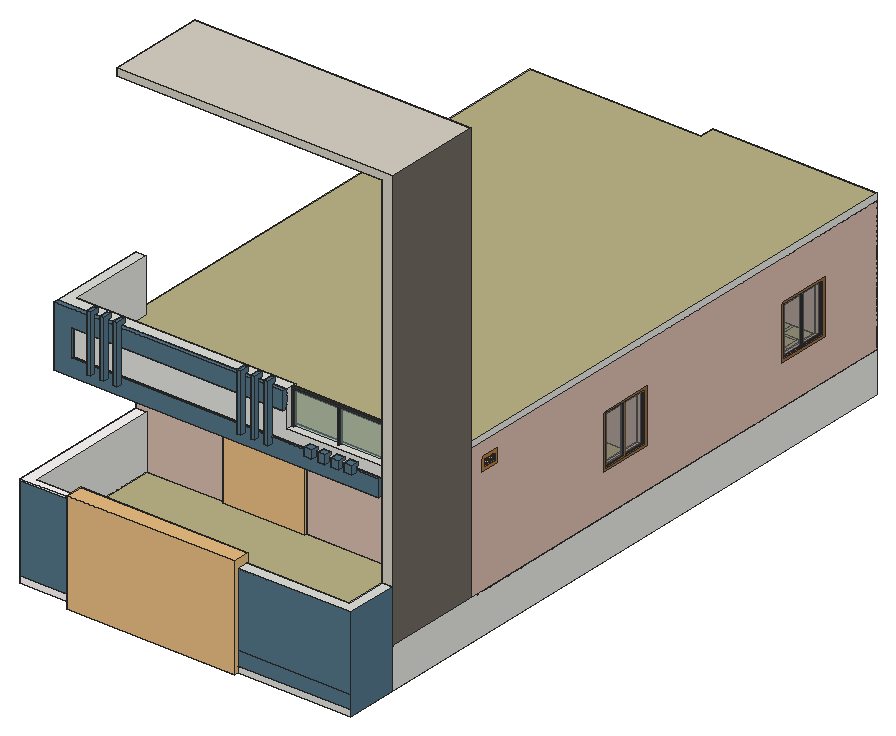
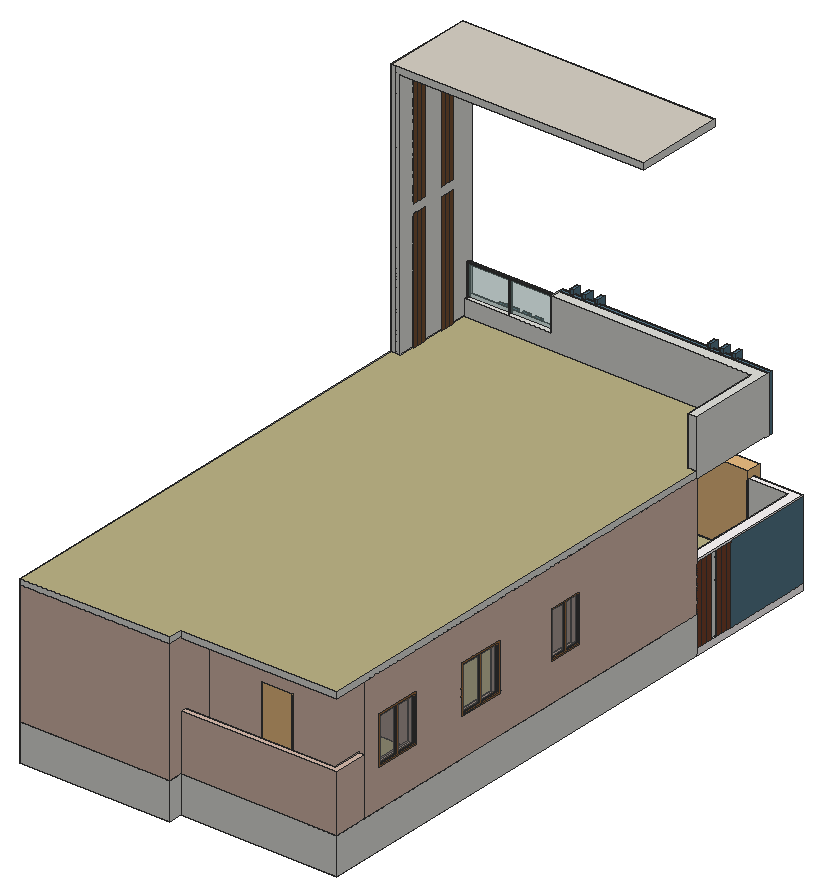
# SketchUp Ruby script. Lengths in inches.
U = 1.inch
M = Sketchup.active_model
def pt(a) = Geom::Point3d.new(a.map { |v| v * U })
def face(e, loops, mat)
  f = e.add_face(loops[0].map { |a| pt(a) })
  loops[1..].each { |l| e.add_face(l.map { |a| pt(a) }).erase! }
  f.material = f.back_material = mat if mat
  f
end
# faces: each face lists its corners as indices into pts; further lists are holes
def faces(e, pts, list, mat = nil) = list.each { |f| face(e, (f[0].is_a?(Array) ? f : [f]).map { |l| l.map { |i| pts[i] } }, mat) }
# xy, xz, yz: faces in a plane at the given z, y or x. An outline is a flat list of corners, or four numbers for a rectangle; further outlines are holes
def ring(l) = l.size == 4 ? [[l[0], l[1]], [l[2], l[1]], [l[2], l[3]], [l[0], l[3]]] : l.each_slice(2).to_a
def flat(e, list, mat, &to3) = list.each { |f| face(e, (f[0].is_a?(Array) ? f : [f]).map { |l| ring(l).map { |u, v| to3.(u, v) } }, mat) }
def xy(e, z, list, mat = nil) = flat(e, list, mat) { |x, y| [x, y, z] }
def xz(e, y, list, mat = nil) = flat(e, list, mat) { |x, z| [x, y, z] }
def yz(e, x, list, mat = nil) = flat(e, list, mat) { |y, z| [x, y, z] }
def lines(e, pts, list) = list.each { |a, b| e.add_line(pt(pts[a]), pt(pts[b])) }
# prism: a flat outline (further loops are holes) pulled along v
def prism(e, loops, v, mat = nil)
  f = face(e, loops, mat); d = Geom::Vector3d.new(v.map { |x| x * U })
  f.pushpull(f.normal.samedirection?(d) ? d.length : -d.length)
end
def box(e, o, s, mat = nil) = prism(e, [[o, [o[0] + s[0], o[1], o[2]], [o[0] + s[0], o[1] + s[1], o[2]], [o[0], o[1] + s[1], o[2]]]], [0, 0, s[2]], mat)
def at(x, y, z, deg = 0) = Geom::Transformation.translation(pt([x, y, z])) * Geom::Transformation.rotation(ORIGIN, Z_AXIS, deg.degrees)
def axes(o, x, y, z) = Geom::Transformation.new([*x, 0, *y, 0, *z, 0, *pt(o).to_a, 1])
def part(name) = M.definitions.add(name)
# library, detail: a bought-in or finely detailed component or shape, given as its bounding box
def library(name, o, s) = part(name).tap { |d| box(d.entities, o, s) }
def detail(e, o, s) = box(e.add_group.entities, o, s)
def put(e, d, t, mat = nil) = e.add_instance(d, t).tap { |i| i.material = mat if mat }
def group(e, t, mat = nil) = e.add_group.tap { |g| g.transformation = t; g.material = mat if mat }.entities
root = M.entities
M.materials.add("TEAKcrown-cut").color = [186, 122, 55]
M.materials.add("[0001_PaleVioletRed]").color = [119, 65, 42]
M.materials.add("[0010_Snow]").color = [255, 250, 250]
M.materials.add("[0027_PeachPuff]").color = [83, 118, 137]
M.materials.add("[0030_OldLace]").color = [216, 209, 197]
M.materials.add("[Carrera Marble]").color = [207, 207, 207]
M.materials.add("[Cladding Weathered]").color = [111, 105, 96]
M.materials.add("[Color B01]").color = [216, 187, 172]
M.materials.add("[Color E03]").color = [255, 255, 101]
M.materials.add("[Color E05]").color = [255, 255, 0]
M.materials.add("[Color M07]").color = [58, 58, 58]
M.materials.add("[Field Rectangle Tile]").color = [193, 186, 176]
M.materials.add("[Sandstone]").color = [118, 81, 52]
M.materials.add("[Stone Marble]").color = [143, 138, 136]
M.materials.add("[Tile Ceramic Natural]").color = [189, 180, 134]
M.materials.add("[Translucent Glass Blue]").color = [141, 178, 174]
M.materials["[Translucent Glass Blue]"].alpha = 0.5
M.materials.add("[Translucent Glass Gray]").color = [128, 128, 128]
M.materials["[Translucent Glass Gray]"].alpha = 0.5
M.materials.add("[Translucent_Glass_Gray]3").color = [255, 255, 255]
M.materials["[Translucent_Glass_Gray]3"].alpha = 0.5
M.materials.add("[Wood Bamboo]").color = [122, 73, 29]
M.materials.add("[Wood Cherry Original]").color = [152, 86, 42]
M.materials.add("[Wood Floor]").color = [155, 105, 61]
c1 = library("Group\#41",[0,0,0],[150.05,15.22,91.0625])
c2 = part("Timber upright")
xy(c2.entities,0,[[0,0,2,5.09]],"[0001_PaleVioletRed]")
xy(c2.entities,76.5,[[0,0,2,5.09]],"[0001_PaleVioletRed]")
xz(c2.entities,0,[[0,0,2,76.5]])
xz(c2.entities,5.09,[[0,0,2,76.5]],"[0001_PaleVioletRed]")
yz(c2.entities,0,[[0,0,5.09,76.5]],"[0001_PaleVioletRed]")
yz(c2.entities,2,[[0,0,5.09,76.5]],"[0001_PaleVioletRed]")
c3 = part("Timber slat")
box(c3.entities,[0,37.3125,0],[3.6875,119.625,1.02],"[Sandstone]")
c4 = part("Group\#44")
put(c4.entities,c3,at(9.375,-37.3125,0))
put(c4.entities,c3,at(4.6875,-37.3125,0))
put(c4.entities,c3,at(0,-37.3125,0))
c5 = library("door by lz",[5.91,-4.92,0],[35.43,6.61,78.74])
c6 = part("Component\#10")
box(c6.entities,[0,0,0],[19,0.25,3.7],"[Translucent_Glass_Gray]3")
c7 = part("Ventilation_window")
g1 = group(c7.entities,at(-76.91,6.38,0),"TEAKcrown-cut")
xy(g1,-1.7,[[0,0,24,3]])
xy(g1,2.5,[[2.5,0,21.5,3]])
xy(g1,17.5,[[2.5,0,21.5,3]])
xy(g1,21.7,[[0,0,24,3]])
xz(g1,0,[[[0,-1.7,24,21.7],[2.5,2.5,21.5,17.5]]],"TEAKcrown-cut")
xz(g1,3,[[[0,-1.7,24,21.7],[2.5,2.5,21.5,17.5]]])
yz(g1,0,[[0,-1.7,3,21.7]])
yz(g1,2.5,[[0,2.5,3,2.5,3,4.31,0,6.48],[3,4.31,3,17.5,0,17.5,0,6.48]])
yz(g1,21.5,[[0,2.5,3,17.5]])
yz(g1,24,[[0,-1.7,3,21.7]])
put(g1,c6,axes([2.5,3.14,11.94],[1,0,0],[0,0.58779,0.80902],[0,-0.80902,0.58779]))
put(g1,c6,axes([2.5,3.16,14.6],[1,0,0],[0,0.58779,0.80902],[0,-0.80902,0.58779]))
put(g1,c6,axes([2.5,3,4.31],[1,0,0],[0,0.58779,0.80902],[0,-0.80902,0.58779]))
put(g1,c6,axes([2.5,3.14,9.46],[1,0,0],[0,0.58779,0.80902],[0,-0.80902,0.58779]))
put(g1,c6,axes([2.5,2.99,7.08],[1,0,0],[0,0.58779,0.80902],[0,-0.80902,0.58779]))
c8 = part("window full")
xy(c8.entities,0,[[0,0,14.17,66.54]])
xy(c8.entities,2.26,[[12.2,2.26,14.17,64.28]],"[Wood Floor]")
xy(c8.entities,2.36,[[0,2.36,1.97,64.17]],"[Wood Floor]")
xy(c8.entities,3.74,[[11.42,3.74,12.2,32.875],[11.42,33.66,12.2,62.79]],"[Wood Floor]")
xy(c8.entities,3.9375,[[1.97,3.9375,2.76,32.77],[1.97,33.76,2.76,62.6]],"[Wood Floor]")
xy(c8.entities,4.18,[[2.76,4.18,11.42,32.09],[2.76,34.45,11.42,62.35]],"[Wood Floor]")
xy(c8.entities,69.83,[[2.76,4.18,11.42,32.09],[2.76,34.45,11.42,62.35]],"[Wood Floor]")
xy(c8.entities,70.08,[[1.97,3.9375,2.76,32.77],[1.97,33.76,2.76,62.6]])
xy(c8.entities,70.27,[[11.42,32.875,12.2,33.66]])
xy(c8.entities,70.27,[[11.42,3.74,12.2,32.875],[11.42,33.66,12.2,62.79]],"[Wood Floor]")
xy(c8.entities,71.65,[[0,2.36,1.97,64.17]])
xy(c8.entities,71.76,[[12.2,2.26,14.17,64.28]],"[Wood Floor]")
xy(c8.entities,74.02,[[0,0,14.17,66.54]],"[Wood Floor]")
xz(c8.entities,0,[[0,0,14.17,74.02]],"[Wood Floor]")
xz(c8.entities,2.26,[[12.2,2.26,14.17,71.76]],"[Wood Floor]")
xz(c8.entities,2.36,[[0,2.36,1.97,71.65]],"[Wood Floor]")
xz(c8.entities,3.74,[[11.42,3.74,12.2,70.27]],"[Wood Floor]")
xz(c8.entities,3.9375,[[1.97,3.9375,2.76,70.08]],"[Wood Floor]")
xz(c8.entities,4.18,[[2.76,4.18,11.42,69.83]],"[Wood Floor]")
xz(c8.entities,32.09,[[2.76,4.18,11.42,69.83]],"[Wood Floor]")
xz(c8.entities,32.77,[[1.97,3.9375,2.76,70.08]],"[Wood Floor]")
xz(c8.entities,32.875,[[11.42,3.74,12.2,70.27]],"[Wood Floor]")
xz(c8.entities,33.66,[[11.42,3.74,12.2,47.88],[11.42,47.88,12.2,70.27]],"[Wood Floor]")
xz(c8.entities,33.76,[[1.97,3.9375,2.76,70.08]],"[Wood Floor]")
xz(c8.entities,34.45,[[2.76,4.18,11.42,69.83]],"[Wood Floor]")
xz(c8.entities,62.35,[[2.76,4.18,11.42,69.83]],"[Wood Floor]")
xz(c8.entities,62.6,[[1.97,3.9375,2.76,70.08]],"[Wood Floor]")
xz(c8.entities,62.79,[[11.42,3.74,12.2,70.27]],"[Wood Floor]")
xz(c8.entities,64.17,[[0,2.36,1.97,71.65]],"[Wood Floor]")
xz(c8.entities,64.28,[[12.2,2.26,14.17,71.76]],"[Wood Floor]")
xz(c8.entities,66.54,[[0,0,14.17,74.02]],"[Wood Floor]")
yz(c8.entities,0,[[[0,0,66.54,74.02],[2.36,2.36,64.17,71.65]]],"[Wood Floor]")
yz(c8.entities,1.97,[[[2.36,2.36,64.17,71.65],[3.9375,3.9375,32.77,70.08],[33.76,3.9375,62.6,70.08]]],"[Wood Floor]")
yz(c8.entities,2.76,[[32.77,3.9375,33.76,4.18],[32.77,4.18,33.76,69.83],[32.77,69.83,33.76,70.08]])
yz(c8.entities,2.76,[[[3.9375,3.9375,32.77,70.08],[4.18,4.18,32.09,69.83]],[[33.76,3.9375,62.6,70.08],[34.45,4.18,62.35,69.83]]],"[Wood Floor]")
yz(c8.entities,11.42,[[32.875,69.83,33.66,70.27]])
yz(c8.entities,11.42,[[[3.74,3.74,32.875,70.27],[4.18,4.18,32.09,69.83]],[[33.66,3.74,62.79,70.27],[34.45,4.18,62.35,69.83]]],"[Wood Floor]")
yz(c8.entities,12.2,[[[2.26,2.26,64.28,71.76],[3.74,3.74,32.875,70.27],[33.66,3.74,62.79,70.27]]],"[Wood Floor]")
yz(c8.entities,14.17,[[[0,0,66.54,74.02],[2.26,2.26,64.28,71.76]]],"[Wood Floor]")
p = [[11.42,32.875,70.27],[11.42,32.875,70.28],[11.42,32.875,69.83],[11.42,32.09,69.83],[11.42,34.45,69.83],[11.42,33.66,69.83]]
lines(c8.entities,p,[[0,1],[2,3],[4,5]])
c9 = part("Group\#7")
g2 = group(c9.entities,at(1.67,3.02,2.71))
yz(g2,0,[[0,0,20.13,42.58]],"[Translucent Glass Gray]")
g3 = group(c9.entities,at(0,0,0))
put(g3,c8,axes([0,0,0],[0.2352,0,0],[0,0.72142,0],[0,0,0.64851]))
g4 = group(g3,at(1.67,24.85,2.71))
yz(g4,0,[[0,0,20.13,42.58]],"[Translucent Glass Gray]")
c10 = part("Group30\#1")
xy(c10.entities,0,[[-14.0625,-20.0625,-0.59,20.0625],[0.59,-20.0625,14.0625,20.0625]],"[Translucent Glass Gray]")
c11 = part("Group29\#1")
prism(c11.entities,[[[-18,24,0],[18,24,0],[18,-24,0],[-18,-24,0]],[[14.0625,20.0625,0],[0.59,20.0625,0],[0.59,-20.0625,0],[14.0625,-20.0625,0]],[[-0.59,20.0625,0],[-14.0625,20.0625,0],[-14.0625,-20.0625,0],[-0.59,-20.0625,0]]],[0,0,5.875],"[Wood Cherry Original]")
put(c11.entities,c10,at(0,0,2.9375))
c12 = part("Union\#2")
xy(c12.entities,0,[[0,87.5,0,494.5,71.05,494.5,71.05,485.5,9,485.5,9,387.5,117,387.5,117,381.5,9,381.5,9,213.5,113.3,213.5,113.3,207.5,9,207.5,9,93.5,79.73,93.5,79.73,87.5],[[153,87.5,153,93.5,239,93.5,239,171.5,153,171.5,153,207.5,143.3,207.5,143.3,213.5,153,213.5,153,286.45,159,286.45,159,177.5,250.23,177.5,250.23,171.5,245,171.5,245,93.5,291,93.5,291,171.5,274.23,171.5,274.23,177.5,291,177.5,291,321.5,159,321.5,159,316.45,153,316.45,153,347.3125,159,347.3125,159,327.5,246,327.5,246,383.5,159,383.5,159,389.5,291,389.5,291,533.5,159,533.5,159,424.27,153,424.27,153,431.5,144.37,431.5,144.37,437.5,153,437.5,153,485.5,117,485.5,117,437.5,124.37,437.5,124.37,431.5,117,431.5,117,424.23,111,424.23,111,485.5,101.05,485.5,101.05,494.5,153,494.5,153,542.5,300,542.5,300,87.5],[252,327.5,291,383.5]],[153,377.3125,158.97,394.27],[111,387.5,117,394.27]])
xy(c12.entities,36,[[250.39,87.5,286.39,93.5],[0,230.6875,9,266.6875],[291,236.77,300,284.77],[0,328.61,9,376.61],[0,430.49,9,478.49],
  [291,436.51,300,484.51]])
xy(c12.entities,84,[[250.39,87.5,286.39,93.5],[250.23,171.5,274.23,177.5],[113.3,207.5,143.3,213.5],[0,230.6875,9,266.6875],[291,236.77,300,284.77],
  [153,286.45,159,316.45],[0,328.61,9,376.61],[153,347.3125,158.97,377.3125],[111,394.27,117,424.23],[153,394.27,159,424.27],
  [0,430.49,9,478.49],[124.37,431.5,144.37,437.5],[291,436.51,300,484.51],[71.05,485.5,101.05,494.5]])
xy(c12.entities,96,[[291,100.54,300,117.47]])
xy(c12.entities,108,[[291,100.54,300,117.47]])
xy(c12.entities,120,[[[0,87.5,79.73,87.5,79.73,93.5,9,93.5,9,207.5,153,207.5,153,171.5,239,171.5,239,93.5,153,93.5,153,87.5,300,87.5,300,542.5,153,542.5,153,494.5,0,494.5],[9,213.5,9,381.5,117,381.5,117,431.5,153,431.5,153,213.5],[159,327.5,159,347.3125,158.97,347.3125,158.97,394.27,159,394.27,159,533.5,291,533.5,291,389.5,159,389.5,159,383.5,246,383.5,246,327.5],[159,177.5,291,321.5],[9,387.5,111,485.5],[245,93.5,291,171.5],[252,327.5,291,383.5],[117,437.5,153,485.5]]])
xz(c12.entities,87.5,[[0,0,79.73,120],[[153,0,300,120],[250.39,36,286.39,84]]])
xz(c12.entities,93.5,[[9,0,79.73,120],[153,0,239,120],[[245,0,291,120],[250.39,36,286.39,84]]])
xz(c12.entities,100.54,[[291,96,300,108]])
xz(c12.entities,117.47,[[291,96,300,108]])
xz(c12.entities,171.5,[[153,0,239,120],[245,0,250.23,0,250.23,84,274.23,84,274.23,0,291,0,291,120,245,120]])
xz(c12.entities,177.5,[[159,0,159,120,291,120,291,0,274.23,0,274.23,84,250.23,84,250.23,0]])
xz(c12.entities,207.5,[[9,0,113.3,0,113.3,84,143.3,84,143.3,0,153,0,153,120,9,120]])
xz(c12.entities,213.5,[[9,0,113.3,120],[143.3,0,143.3,84,113.3,84,113.3,120,153,120,153,0]])
xz(c12.entities,230.6875,[[0,36,9,84]])
xz(c12.entities,236.77,[[291,36,300,84]])
xz(c12.entities,266.6875,[[0,36,9,84]])
xz(c12.entities,284.77,[[291,36,300,84]])
xz(c12.entities,286.45,[[153,0,159,84]])
xz(c12.entities,316.45,[[153,0,159,84]])
xz(c12.entities,321.5,[[159,0,291,120]])
xz(c12.entities,327.5,[[159,0,246,120],[252,0,291,120]])
xz(c12.entities,328.61,[[0,36,9,84]])
xz(c12.entities,347.3125,[[153,0,153,84,158.97,84,158.97,120,159,120,159,0]])
xz(c12.entities,376.61,[[0,36,9,84]])
xz(c12.entities,377.3125,[[153,0,158.97,84]])
xz(c12.entities,381.5,[[9,0,117,120]])
xz(c12.entities,383.5,[[159,0,246,120],[252,0,291,120]])
xz(c12.entities,387.5,[[9,0,111,120]])
xz(c12.entities,389.5,[[159,0,291,120]])
xz(c12.entities,394.27,[[111,0,117,84],[153,0,158.97,84],[158.97,84,159,120]])
xz(c12.entities,424.23,[[111,0,117,84]])
xz(c12.entities,424.27,[[153,0,159,84]])
xz(c12.entities,430.49,[[0,36,9,84]])
xz(c12.entities,431.5,[[117,0,124.37,0,124.37,84,144.37,84,144.37,0,153,0,153,120,117,120]])
xz(c12.entities,436.51,[[291,36,300,84]])
xz(c12.entities,437.5,[[117,0,117,120,153,120,153,0,144.37,0,144.37,84,124.37,84,124.37,0]])
xz(c12.entities,478.49,[[0,36,9,84]])
xz(c12.entities,484.51,[[291,36,300,84]])
xz(c12.entities,485.5,[[9,0,71.05,0,71.05,84,101.05,84,101.05,0,111,0,111,120,9,120],[117,0,153,120]])
xz(c12.entities,494.5,[[0,0,0,120,153,120,153,0,101.05,0,101.05,84,71.05,84,71.05,0]])
xz(c12.entities,533.5,[[159,0,291,120]])
xz(c12.entities,542.5,[[153,0,300,120]])
yz(c12.entities,0,[[[87.5,0,494.5,120],[430.49,36,478.49,84],[328.61,36,376.61,84],[230.6875,36,266.6875,84]]])
yz(c12.entities,9,[[93.5,0,207.5,120],[[213.5,0,381.5,120],[328.61,36,376.61,84],[230.6875,36,266.6875,84]],[[387.5,0,485.5,120],[430.49,36,478.49,84]]])
yz(c12.entities,71.05,[[485.5,0,494.5,84]])
yz(c12.entities,79.73,[[87.5,0,93.5,120]])
yz(c12.entities,101.05,[[485.5,0,494.5,84]])
yz(c12.entities,111,[[387.5,0,387.5,120,485.5,120,485.5,0,424.23,0,424.23,84,394.27,84,394.27,0]])
yz(c12.entities,113.3,[[207.5,0,213.5,84]])
yz(c12.entities,117,[[381.5,0,394.27,0,394.27,84,424.23,84,424.23,0,431.5,0,431.5,120,381.5,120],[437.5,0,485.5,120]])
yz(c12.entities,124.37,[[431.5,0,437.5,84]])
yz(c12.entities,143.3,[[207.5,0,213.5,84]])
yz(c12.entities,144.37,[[431.5,0,437.5,84]])
yz(c12.entities,153,[[87.5,0,93.5,120],[171.5,0,207.5,120],[213.5,0,213.5,120,431.5,120,431.5,0,424.27,0,424.27,84,394.27,84,394.27,0,377.3125,0,377.3125,84,347.3125,84,347.3125,0,316.45,0,316.45,84,286.45,84,286.45,0],[437.5,0,485.5,120],[494.5,0,542.5,120]])
yz(c12.entities,158.97,[[377.3125,0,394.27,0,394.27,120,347.3125,120,347.3125,84,377.3125,84]])
yz(c12.entities,159,[[177.5,0,286.45,0,286.45,84,316.45,84,316.45,0,321.5,0,321.5,120,177.5,120],[327.5,0,347.3125,120],[383.5,0,389.5,120],[424.27,0,533.5,0,533.5,120,394.27,120,394.27,84,424.27,84]])
yz(c12.entities,239,[[93.5,0,171.5,120]])
yz(c12.entities,245,[[93.5,0,171.5,120]])
yz(c12.entities,246,[[327.5,0,383.5,120]])
yz(c12.entities,250.23,[[171.5,0,177.5,84]])
yz(c12.entities,250.39,[[87.5,36,93.5,84]])
yz(c12.entities,252,[[327.5,0,383.5,120]])
yz(c12.entities,274.23,[[171.5,0,177.5,84]])
yz(c12.entities,286.39,[[87.5,36,93.5,84]])
yz(c12.entities,291,[[[93.5,0,171.5,120],[100.54,96,117.47,108]],[[177.5,0,321.5,120],[236.77,36,284.77,84]],[327.5,0,383.5,120],[[389.5,0,533.5,120],[436.51,36,484.51,84]]])
yz(c12.entities,300,[[[87.5,0,542.5,120],[436.51,36,484.51,84],[236.77,36,284.77,84],[100.54,96,117.47,108]]])
put(c12.entities,c5,axes([153.59,321.46,0],[0,-0.84667,0],[0.14881,0,0],[0,0,1.0668]))
put(c12.entities,c5,axes([153.59,382.32,0],[0,-0.84667,0],[0.14881,0,0],[0,0,1.0668]))
put(c12.entities,c5,axes([153.59,429.27,0],[0,-0.84667,0],[0.14881,0,0],[0,0,1.0668]))
put(c12.entities,c5,axes([116.41,429.27,0],[0,-0.84667,0],[-0.14881,0,0],[0,0,1.0668]))
put(c12.entities,c5,axes([108.3,208.09,0],[0.84667,0,0],[0,0.14881,0],[0,0,1.0668]))
put(c12.entities,c5,axes([246.23,177.5,0],[0.67733,0,0],[0,0.14881,0],[0,0,1.0668]))
put(c12.entities,c5,axes([66.05,494.59,0],[0.84667,0,0],[0,0.14881,0],[0,0,1.0668]))
put(c12.entities,c7,axes([303.45,154.81,96.87],[0,0.70573,0],[-0.54,0,0],[0,0,0.51282]))
put(c12.entities,c9,at(0,328.61,36))
put(c12.entities,c9,at(0,430.49,36))
put(c12.entities,c9,at(296.67,436.51,36))
put(c12.entities,c9,at(296.67,236.77,36))
put(c12.entities,c9,axes([0,230.6875,36],[1,0,0],[0,0.75,0],[0,0,1]))
put(c12.entities,c11,axes([268.39,93.375,60],[1,0,0],[0,0,1],[0,-1,0]))
c13 = library("Group\#49",[0,0,0],[78.74,4.71,80.71])
c14 = part("Bed - Queen")
p = [[22,23.6,0],[16.8,23.6,0],[22,38.8,0],[1.2,38.8,0],[1.2,25.6,0],[-1.2,38.8,0],
  [-1.2,25.6,0],[-22,38.8,0],[-22,25.6,0],[30,-40,0],[-30,-40,0],[-30,40,0],
  [14.8,23.2,0],[-30,23.2,0],[-30,25.6,0],[14.8,25.6,0],[30,40,0],[30,10.4,0],
  [14.8,10.4,0]]
lines(c14.entities,p,[[0,1],[2,0],[3,2],[4,3],[5,6],[7,5],[8,7],[9,10],[10,11],[12,13],[14,15],[11,16],
  [16,9],[17,15],[18,17],[15,18]])
c15 = library("*U5",[-21.75,-46.5,0],[21,33,0.01])
c16 = part("*U1")
p = [[-20,-17,0],[-20,23,0],[-18.25,23,0],[-18.25,-17,0],[20,-17,0],[19.92,-14.49,0],
  [19.68,-11.99,0],[19.29,-9.5,0],[18.74,-7.05,0],[18.04,-4.64,0],[17.19,-2.28,0],[16.19,0.03,0],
  [15.05,2.27,0],[13.77,4.43,0],[12.36,6.51,0],[10.82,8.5,0],[9.16,10.38,0],[7.38,12.16,0],
  [5.5,13.82,0],[3.51,15.36,0],[1.43,16.77,0],[-0.73,18.05,0],[-2.97,19.19,0],[-5.28,20.19,0],
  [-7.64,21.04,0],[-10.05,21.74,0],[-12.5,22.29,0],[-14.99,22.68,0],[-17.49,22.92,0],[-20,-23,0],
  [20,-23,0]]
lines(c16.entities,p,[[0,1],[1,2],[2,3],[3,0],[4,5],[5,6],[6,7],[7,8],[8,9],[9,10],[10,11],[11,12],
  [12,13],[13,14],[14,15],[15,16],[16,17],[17,18],[18,19],[19,20],[20,21],[21,22],[22,23],[23,24],
  [24,25],[25,26],[26,27],[27,28],[28,1],[0,29],[4,30]])
c17 = library("SINK",[-14.49,-22.42,0],[28.98,44.84,0.01])
c18 = library("new block",[-14.35,-4.62,0],[28.7,9.24,0.01])
c19 = part("Union\#4")
prism(c19.entities,[[[153,29,0],[6,29,0],[6,0,0],[0,0,0],[0,35,0],[153,35,0]]],[0,0,55.4375])
c20 = library("Group\#3",[0,0,0],[86,78,119.99])
c21 = part("Component\#9")
xy(c21.entities,0,[[[0,0,6.875,4],[0.7,0.7,6.17,3.3]]],"[Color E05]")
xy(c21.entities,0.625,[[0.7,0.7,6.17,3.3]],"[Color E05]")
xy(c21.entities,4.5625,[[0,4,6.875,6.6875]])
xy(c21.entities,7.25,[[0,0,6.875,6.6875]],"[0027_PeachPuff]")
xz(c21.entities,0,[[0,0,6.875,7.25]],"[0027_PeachPuff]")
xz(c21.entities,0.7,[[0.7,0,6.17,0.625]])
xz(c21.entities,3.3,[[0.7,0,6.17,0.625]],"[Color E05]")
xz(c21.entities,4,[[0,0,6.875,4.5625]])
xz(c21.entities,6.6875,[[0,4.5625,6.875,7.25]])
yz(c21.entities,0,[[0,0,0,7.25,6.6875,7.25,6.6875,4.5625,4,4.5625,4,0]],"[0027_PeachPuff]")
yz(c21.entities,0.7,[[0.7,0,3.3,0.625]],"[Color E05]")
yz(c21.entities,6.17,[[0.7,0,3.3,0.625]],"[Color E05]")
yz(c21.entities,6.875,[[0,0,4,0,4,4.5625,6.6875,4.5625,6.6875,7.25,0,7.25]],"[0027_PeachPuff]")
c22 = part("Vertical support post")
prism(c22.entities,[[[3.5625,0,-4],[3.5625,0,43.375],[3.5625,4,43.375],[3.5625,4,47.375],[3.5625,-4,47.375],[3.5625,-4,-4]]],[-3.5625,0,0],"[0027_PeachPuff]")
c23 = part("Group70\#1")
box(c23.entities,[313.8,73.72,268.25],[1.18,2.36,29.23])
c24 = part("Group69\#1")
box(c24.entities,[356.12,73.72,268.25],[2.36,2.36,29.23])
c25 = part("Group71\#1")
box(c25.entities,[270.3,73.52,297.48],[88.18,2.76,1.77])
c26 = part("Group68\#1")
box(c26.entities,[270.3,73.72,268.25],[2.37,2.36,29.23])
c27 = part("Group74\#1")
xz(c27.entities,74.9,[[271.49,268.25,357.3,297.48]],"[Translucent Glass Blue]")
c28 = part("Group\#12")
put(c28.entities,c23,at(-270.3,-73.52,-268.25),"[Color M07]")
put(c28.entities,c24,at(-270.3,-73.52,-268.25),"[Color M07]")
put(c28.entities,c25,at(-270.3,-73.52,-268.25),"[Color M07]")
put(c28.entities,c26,at(-270.3,-73.52,-268.25),"[Color M07]")
put(c28.entities,c27,at(-270.3,-73.52,-268.25))
xy(root,29.75,[[291,134.5,300,147.55],[159,368.5,291,368.5,291,374.5,252,374.5,252,396.64,246,396.64,246,374.5,159,374.5],[0,375.61,3.35,423.61],[3.35,375.61,5.29,423.61],[5.29,375.61,9,423.61],
  [153,394.3125,159,394.3125,159,394.35],[246,408.36,252,408.36,252,436.5,159,436.5,159,430.5,246,430.5],[153,441.27,159,442.58],[153,471.27,159,471.27,159,580.5,153,580.5,153,484.5,144.37,484.5,144.37,478.5,153,478.5],[0,477.49,3.35,525.49],
  [3.35,477.49,5.29,525.49],[5.29,477.49,9,525.49],[121.26,532.5,136.71,535.82],[121.26,535.82,136.71,537.92],[121.26,537.92,136.71,540.72],
  [6,541.5,153,570.5]])
xy(root,83.0625,[[49.61,0,63.63,9.98]],"[Field Rectangle Tile]")
p = [[117,471.23,29.75],[117,478.5,29.75],[153,176.5,29.75],[153,182.5,29.75],[163.19,176.5,29.75],[300,331.77,29.75],
  [300,483.51,29.75],[178.26,197.66,29.75],[183.1,197.66,29.75],[153,394.3125,29.75],[153,424.3125,29.75],[296.37,164.47,29.75],
  [300,164.47,29.75],[300,531.51,29.75],[173.15,176.5,29.75],[300,283.77,29.75],[193.05,197.66,29.75],[197.3125,197.66,29.75],
  [291,224.5,29.75],[291,283.77,29.75],[153,197.66,29.75],[300,147.55,29.75],[296.29,331.77,29.75],[291,436.5,29.75],
  [291,483.51,29.75],[198.7,197.66,29.75],[203,197.66,29.75],[193.05,218.5,29.75],[203,218.5,29.75],[4.43,313.6875,29.75],
  [5.55,313.6875,29.75],[209,197.66,29.75],[257.37,434.17,29.75],[257.37,436.25,29.75],[0,375.61,29.75],[0,313.6875,29.75],
  [153,260.5,29.75],[153,333.45,29.75],[296.29,531.51,29.75],[0,277.6875,29.75],[-0.07,277.6875,29.75],[203,140.5,29.75],
  [239,140.5,29.75],[291,331.77,29.75],[291,368.5,29.75],[176.88,197.66,29.75],[153,363.45,29.75],[291,374.5,29.75],
  [291,430.5,29.75],[163.19,197.66,29.75],[173.15,197.66,29.75],[300,589.5,29.75],[153,442.58,29.75],[153,471.27,29.75],
  [291,531.51,29.75],[291,580.5,29.75],[160.46,197.66,29.75],[161.85,197.66,29.75],[0,178.14,29.75],[9,178.14,29.75],
  [257.37,433.49,29.75],[257.37,372.24,29.75],[257.37,374.3125,29.75],[257.37,371.55,29.75],[163.19,182.5,29.75],[8.93,313.6875,29.75],
  [239,218.5,29.75],[183.1,218.5,29.75],[246,396.64,29.75],[245.77,396.64,29.75],[173.15,182.5,29.75],[0,477.49,29.75],
  [0,423.61,29.75],[210.39,197.66,29.75],[212.78,197.66,29.75],[153,254.5,29.75],[111,434.5,29.75],[111,442.58,29.75],
  [111,471.23,29.75],[111,532.5,29.75],[159,471.23,29.75],[159,471.27,29.75],[159,224.5,29.75],[159,333.45,29.75],
  [245,140.5,29.75],[245,218.5,29.75],[117,428.5,29.75],[117,434.5,29.75],[239,141.85,29.75],[153,134.5,29.75],
  [291,134.5,29.75],[153,140.5,29.75],[163.19,140.5,29.75],[117,484.5,29.75],[117,532.5,29.75],[193.05,176.5,29.75],
  [193.05,163.64,29.75],[101.05,541.5,29.75],[101.05,532.5,29.75],[274.23,218.5,29.75],[291,218.5,29.75],[97,254.5,29.75],
  [97,218.5,29.75],[193.05,182.5,29.75],[163.19,163.64,29.75],[203.02,178.29,29.75],[212.78,168.41,29.75],[212.78,163.64,29.75],
  [207.17,163.64,29.75],[160.46,196.47,29.75],[160.46,198.47,29.75],[113.34,260.5,29.75],[113.3,260.5,29.75],[9,428.5,29.75],
  [139.62,250.68,29.75],[134.2,254.5,29.75],[176.88,198.47,29.75],[203,179.5,29.75],[212.78,190.1,29.75],[209,198.47,29.75],
  [209,196.47,29.75],[250.23,218.5,29.75],[197.3125,198.47,29.75],[183.1,182.5,29.75],[203,176.5,29.75],[203,163.64,29.75],
  [156.46,162.64,29.75],[156.46,163.64,29.75],[117,254.5,29.75],[117,218.5,29.75],[239,179.5,29.75],[212.78,179.5,29.75],
  [155.08,163.46,29.75],[113.3,254.5,29.75],[153,218.5,29.75],[163.19,218.5,29.75],[169.98,162.64,29.75],[169.98,163.64,29.75],
  [252,430.5,29.75],[107,254.5,29.75],[107,218.5,29.75],[173.15,163.64,29.75],[146.69,197.66,29.75],[176.88,196.47,29.75],
  [250.23,224.5,29.75],[197.3125,196.47,29.75],[274.23,224.5,29.75],[153,589.5,29.75],[159,589.5,29.75],[156.46,164.64,29.75],
  [155.29,163.64,29.75],[129.625,250.68,29.75],[291,140.5,29.75],[183.1,176.5,29.75],[183.1,163.64,29.75],[203,182.5,29.75],
  [207.17,162.64,29.75],[296.29,483.51,29.75],[187.2,164.64,29.75],[186.03,163.64,29.75],[294.35,531.51,29.75],[4.43,277.6875,29.75],
  [279.48,371.55,29.75],[-0.07,313.6875,29.75],[32.58,506.5,29.75],[32.58,434.5,29.75],[168.59,163.46,29.75],[207.17,164.64,29.75],
  [206,163.64,29.75],[294.35,483.51,29.75],[65.91,532.5,29.75],[65.91,530.5,29.75],[187.2,162.64,29.75],[187.2,163.64,29.75],
  [5.55,277.6875,29.75],[279.48,372.24,29.75],[279.48,436.25,29.75],[279.48,434.17,29.75],[296.29,283.77,29.75],[279.48,430.72,29.75],
  [257.37,430.72,29.75],[257.37,432.58,29.75],[279.48,432.58,29.75],[279.48,433.49,29.75],[205.78,163.46,29.75],[271.5,402.5,29.75],
  [123.69,478.5,29.75],[123.69,484.5,29.75],[117,442.58,29.75],[8.93,277.6875,29.75],[257.37,370.64,29.75],[279.48,370.64,29.75],
  [264.27,164.4,29.75],[264.27,164.54,29.75],[264.26,164.67,29.75],[65.91,506.5,29.75],[279.48,368.79,29.75],[257.37,368.79,29.75],
  [185.82,163.46,29.75],[294.35,331.77,29.75],[169.98,164.64,29.75],[168.81,163.64,29.75],[2.95,313.6875,29.75],[2.95,277.6875,29.75],
  [279.48,374.3125,29.75],[294.35,283.77,29.75],[262.87,166.37,29.75],[262.74,166.41,29.75],[263.35,166.13,29.75],[263.24,166.2,29.75],
  [260.28,163.61,29.75],[260.34,163.48,29.75],[260.93,166.05,29.75],[260.83,165.96,29.75],[260.64,165.77,29.75],[260.55,165.67,29.75],
  [260.28,165.2,29.75],[260.23,165.07,29.75],[260.4,163.36,29.75],[260.47,163.25,29.75],[260.55,163.14,29.75],[264.23,164.81,29.75],
  [264.2,164.9375,29.75],[262.6,166.4375,29.75],[262.47,166.46,29.75],[260.64,163.03,29.75],[260.73,162.93,29.75],[263.67,165.87,29.75],
  [263.57,165.96,29.75],[261.53,166.37,29.75],[261.4,166.32,29.75],[264.12,165.2,29.75],[264.06,165.32,29.75],[264,165.44,29.75],
  [263.92,165.56,29.75],[260.19,164.9375,29.75],[261.04,166.13,29.75],[260.14,164.67,29.75],[260.125,164.54,29.75],[260.125,164.27,29.75],
  [260.14,164.13,29.75],[263.46,166.05,29.75],[262.99,166.32,29.75],[260.34,165.32,29.75],[260.73,165.87,29.75],[260.12,164.4,29.75],
  [260.47,165.56,29.75],[260.16,164,29.75],[264.16,165.07,29.75],[261.28,166.26,29.75],[261.16,166.2,29.75],[260.19,163.86,29.75],
  [260.83,162.84,29.75],[260.93,162.76,29.75],[261.04,162.68,29.75],[263.12,166.26,29.75],[261.16,162.6,29.75],[260.16,164.81,29.75],
  [261.28,162.54,29.75],[261.4,162.48,29.75],[262.33,166.47,29.75],[262.2,166.48,29.75],[261.93,166.46,29.75],[261.79,166.4375,29.75],
  [263.76,165.77,29.75],[261.66,166.41,29.75],[263.85,165.67,29.75],[260.4,165.44,29.75],[260.23,163.73,29.75],[262.0625,166.47,29.75],
  [264.06,163.48,29.75],[264.12,163.61,29.75],[262.6,162.37,29.75],[262.74,162.4,29.75],[223.78,404.26,29.75],[223.69,404.35,29.75],
  [261.53,162.4375,29.75],[261.66,162.4,29.75],[224.37,402.96,29.75],[224.36,403.09,29.75],[263.35,162.68,29.75],[263.46,162.76,29.75],
  [223.96,404.06,29.75],[223.87,404.16,29.75],[223.58,404.43,29.75],[223.25,404.64,29.75],[223.125,404.7,29.75],[223.47,404.51,29.75],
  [223.36,404.58,29.75],[223,404.74,29.75],[222.875,404.78,29.75],[222.74,404.81,29.75],[263.92,163.25,29.75],[264,163.36,29.75],
  [222.35,404.85,29.75],[222.22,404.85,29.75],[262.47,162.34,29.75],[224.34,403.22,29.75],[224.31,403.35,29.75],[222.08,404.83,29.75],
  [221.95,404.81,29.75],[221.82,404.78,29.75],[263.85,163.14,29.75],[264.27,164.27,29.75],[262.87,162.4375,29.75],[224.22,403.6,29.75],
  [224.17,403.72,29.75],[222.61,404.83,29.75],[264.23,164,29.75],[264.26,164.13,29.75],[263.57,162.84,29.75],[221.7,404.74,29.75],
  [221.57,404.7,29.75],[221.45,404.64,29.75],[224.27,403.47,29.75],[222.48,404.85,29.75],[264.16,163.73,29.75],[224.03,403.95,29.75],
  [221.34,404.58,29.75],[221.22,404.51,29.75],[221.12,404.43,29.75],[224.1,403.84,29.75],[261.93,162.34,29.75],[262.0625,162.33,29.75],
  [261.79,162.37,29.75],[262.2,162.33,29.75],[262.33,162.33,29.75],[262.99,162.48,29.75],[263.12,162.54,29.75],[263.76,163.03,29.75],
  [264.2,163.86,29.75],[224.375,402.82,29.75],[263.24,162.6,29.75],[263.67,162.93,29.75],[223.58,401.22,29.75],[223.69,401.3,29.75],
  [220.59,403.84,29.75],[220.53,403.72,29.75],[221.22,401.14,29.75],[221.34,401.07,29.75],[221.7,400.9,29.75],[221.82,400.87,29.75],
  [223.78,401.39,29.75],[223.87,401.49,29.75],[223.96,401.59,29.75],[224.17,401.93,29.75],[224.22,402.05,29.75],[224.31,402.3,29.75],
  [224.34,402.43,29.75],[224.27,402.17,29.75],[224.36,402.56,29.75],[291,164.47,29.75],[294.07,164.47,29.75],[220.83,404.16,29.75],
  [220.74,404.06,29.75],[220.33,402.96,29.75],[220.32,402.82,29.75],[220.48,402.05,29.75],[220.53,401.93,29.75],[220.74,401.59,29.75],
  [220.83,401.49,29.75],[221.95,400.84,29.75],[220.48,403.6,29.75],[222.22,400.8,29.75],[222.35,400.8,29.75],[222.48,400.8,29.75],
  [222.61,400.8125,29.75],[220.66,403.95,29.75],[222.74,400.84,29.75],[220.66,401.7,29.75],[221.57,400.95,29.75],[222.875,400.87,29.75],
  [220.39,403.35,29.75],[220.36,403.22,29.75],[223,400.9,29.75],[220.59,401.81,29.75],[223.125,400.95,29.75],[223.47,401.14,29.75],
  [221.01,401.3,29.75],[221.12,401.22,29.75],[224.03,401.7,29.75],[220.43,403.47,29.75],[224.1,401.81,29.75],[224.37,402.69,29.75],
  [222.08,400.8125,29.75],[220.33,402.69,29.75],[221.45,401.01,29.75],[220.36,402.43,29.75],[220.39,402.3,29.75],[220.43,402.17,29.75],
  [220.92,404.26,29.75],[220.92,401.39,29.75],[223.25,401.01,29.75],[221.01,404.35,29.75],[223.36,401.07,29.75],[220.34,402.56,29.75],
  [220.34,403.09,29.75],[159,580.5,29.75],[71.05,532.5,29.75],[252,436.5,29.75],[9,254.5,29.75],[9,434.5,29.75],
  [143.3,254.5,29.75],[9,260.5,29.75],[9,477.49,29.75],[245.77,408.36,29.75],[9,423.61,29.75],[136.71,532.5,29.75],
  [153,532.5,29.75],[252,396.64,29.75],[252,408.36,29.75],[183.1,140.5,29.75],[193.05,140.5,29.75],[9,532.5,29.75],
  [173.15,218.5,29.75],[246,408.36,29.75],[9,541.5,29.75],[296.37,147.55,29.75],[249.48,408.36,29.75],[249.48,396.64,29.75],
  [121.26,532.5,29.75],[159,333.49,29.75],[71.05,541.5,29.75],[9,525.49,29.75],[294.07,147.55,29.75],[247.89,396.64,29.75],
  [247.89,408.36,29.75],[9,375.61,29.75],[173.15,140.5,29.75],[144.37,478.5,29.75],[144.37,484.5,29.75],[153,163.64,29.75],
  [146.69,163.64,29.75],[252,374.5,29.75],[0,541.5,29.75],[0,525.49,29.75],[291,147.55,29.75],[240.31,140.52,29.75],
  [153,580.5,29.75],[200.65,0,-1],[197.65,0,-1]]
lines(root,p,[[0,1],[2,3],[4,2],[5,6],[7,8],[9,10],[11,12],[6,13],[14,4],[15,5],[16,17],[18,19],
  [3,20],[21,12],[22,5],[23,24],[25,26],[17,25],[27,28],[29,30],[8,16],[26,31],[32,33],[34,35],
  [36,37],[38,13],[39,40],[41,42],[43,44],[45,7],[37,46],[47,48],[49,50],[48,23],[35,39],[13,51],
  [52,53],[54,55],[12,15],[24,54],[56,57],[58,59],[60,32],[61,62],[19,43],[63,61],[39,58],[64,3],
  [30,65],[50,45],[28,66],[67,27],[68,69],[70,64],[71,72],[31,73],[73,74],[36,75],[76,77],[78,79],
  [80,81],[82,83],[84,85],[86,87],[42,88],[89,90],[91,92],[93,94],[95,96],[97,98],[70,50],[99,100],
  [101,102],[103,16],[4,104],[105,106],[107,108],[109,57],[57,110],[111,112],[86,113],[114,115],[116,45],[117,118],
  [119,31],[120,73],[85,121],[122,17],[123,8],[124,125],[126,127],[128,129],[130,131],[74,118],[132,126],[133,112],
  [134,135],[136,137],[64,49],[124,117],[25,122],[73,119],[138,48],[139,140],[14,141],[37,83],[142,20],[143,7],
  [121,144],[102,140],[145,25],[146,99],[147,148],[110,56],[7,116],[149,150],[151,114],[84,152],[153,154],[87,76],
  [82,144],[115,151],[155,103],[124,95],[156,108],[157,38],[158,159],[54,160],[161,29],[162,63],[40,163],[164,165],
  [166,136],[167,168],[160,169],[170,171],[172,173],[30,174],[61,175],[176,177],[15,178],[179,180],[181,182],[183,60],
  [184,156],[138,185],[48,185],[186,187],[77,188],[189,174],[78,0],[190,191],[192,193],[65,189],[193,194],[171,195],
  [196,197],[180,181],[195,164],[198,172],[43,199],[163,35],[200,201],[202,203],[197,190],[62,204],[204,175],[199,205],
  [178,22],[33,176],[32,177],[6,157],[206,207],[208,209],[210,211],[212,213],[214,215],[216,217],[218,219],[219,220],
  [221,222],[223,224],[220,225],[225,226],[227,228],[229,230],[231,232],[233,234],[217,235],[236,212],[237,238],[239,240],
  [228,241],[242,206],[243,216],[244,214],[245,239],[215,246],[240,247],[248,231],[249,250],[247,251],[222,248],[211,218],
  [226,252],[252,253],[253,254],[209,255],[254,256],[235,257],[256,258],[258,259],[224,260],[260,261],[262,263],[232,233],
  [264,227],[263,265],[255,242],[207,223],[266,264],[246,267],[238,245],[267,243],[251,268],[268,210],[241,208],[269,262],
  [230,249],[261,269],[250,236],[213,244],[234,266],[194,221],[265,229],[257,237],[270,271],[272,273],[274,275],[276,277],
  [278,279],[280,281],[282,283],[275,284],[283,274],[285,286],[287,288],[289,290],[288,285],[290,291],[292,293],[286,289],
  [294,295],[296,272],[297,298],[299,300],[300,301],[302,292],[303,192],[273,304],[305,306],[291,307],[308,309],[281,310],
  [301,311],[312,313],[293,270],[314,305],[307,315],[259,276],[309,303],[279,297],[311,312],[271,316],[317,282],[295,299],
  [313,318],[319,320],[321,317],[315,294],[318,319],[322,323],[324,322],[325,326],[327,328],[329,302],[316,330],[284,287],
  [304,327],[330,308],[331,278],[298,314],[277,324],[306,321],[328,332],[310,333],[326,296],[323,325],[332,280],[333,329],
  [334,335],[336,337],[338,339],[340,341],[342,343],[343,344],[345,346],[347,348],[349,347],[348,350],[351,352],[353,354],
  [355,356],[357,358],[359,360],[341,361],[337,362],[363,364],[365,366],[354,367],[366,368],[369,359],[370,340],[368,371],
  [372,373],[371,374],[375,369],[374,376],[377,334],[335,342],[378,379],[344,380],[362,381],[380,382],[350,383],[383,331],
  [361,384],[346,349],[379,338],[356,385],[339,386],[387,388],[388,389],[390,353],[391,378],[376,392],[382,345],[393,390],
  [364,365],[360,391],[386,370],[392,394],[394,377],[367,336],[395,387],[396,355],[385,395],[358,375],[384,363],[320,393],
  [381,372],[373,396],[389,357],[397,55],[398,98],[399,23],[101,400],[98,79],[113,401],[139,101],[402,115],[112,403],
  [76,165],[400,403],[87,188],[401,404],[69,405],[406,113],[407,408],[409,410],[130,66],[411,412],[413,170],[135,414],
  [148,51],[405,415],[413,416],[11,417],[89,91],[418,419],[59,400],[94,420],[170,398],[83,421],[422,398],[68,415],
  [88,130],[423,413],[79,94],[424,352],[425,426],[403,427],[428,411],[92,428],[144,146],[49,135],[118,131],[141,137],
  [50,414],[140,129],[173,159],[56,109],[201,104],[31,120],[173,158],[125,41],[108,167],[150,132],[45,143],[201,166],
  [168,184],[187,93],[155,26],[117,155],[106,107],[131,106],[127,149],[429,186],[127,150],[205,19],[96,173],[125,96],
  [178,205],[430,187],[159,198],[96,412],[8,67],[199,22],[160,38],[169,24],[159,154],[157,169],[103,123],[141,428],
  [137,200],[154,411],[131,117],[118,66],[16,27],[106,88],[431,432],[104,127],[150,431],[17,145],[95,153],[137,201],
  [108,168],[20,56],[104,92],[154,141],[168,125],[431,2],[203,39],[186,1],[183,182],[185,47],[129,134],[185,433],
  [133,139],[20,134],[434,435],[26,28],[91,431],[412,41],[191,196],[174,161],[146,18],[153,14],[190,63],[188,0],
  [436,351],[123,70],[88,437],[57,49],[351,100],[100,18],[181,60],[134,75],[175,162],[438,147],[162,191],[177,183],
  [165,401],[161,203],[182,179],[35,202],[352,11],[414,67],[397,148],[128,133],[115,128],[202,29],[439,440]])
g5 = group(root,at(0,47,23.75))
xy(g5,-30,[[197.65,-47,197.65,-37.02,49.26,-37.02,49.26,-36.01,10.08,-36.01,10.08,87.5,0,87.5,0,529.5,153,529.5,153,542.5,300,542.5,300,-47]])
xy(g5,-21,[[63.63,-37.02,183.63,-27.02]],"[Stone Marble]")
xy(g5,-12,[[63.63,-27.02,183.63,-20.5]],"[Stone Marble]")
xy(g5,-3,[[63.63,-20.5,183.63,-10]],"[Stone Marble]")
xy(g5,6,[[49.26,-37.02,63.63,-37.02,63.63,-10,183.63,-10,183.63,-37.02,291,-37.02,291,0,300,0,300,542.5,153,542.5,153,529.5,0,529.5,0,87.5,10.08,87.5,10.08,-36.01,49.26,-36.01]],"[Tile Ceramic Natural]")
xy(g5,54,[[197.65,-47,300,-47,300,0,291,0,291,-37.02,197.65,-37.02]])
xz(g5,-47,[[197.65,-30,300,-30,300,-24.75,198.4,-24.75,198.4,-12,197.65,-12],[197.65,-12,198.4,54]])
xz(g5,-47,[[198.4,-24.75,300,-12],[198.4,-12,300,54]],"[0027_PeachPuff]")
xz(g5,-37.02,[[49.26,-30,63.63,6],[183.63,-30,197.65,-12],[183.63,-12,197.65,6],[197.65,6,291,54]])
xz(g5,-37.02,[[63.63,-30,183.63,-21]],"[Stone Marble]")
xz(g5,-36.01,[[10.08,-30,49.26,6]])
xz(g5,-27.02,[[63.63,-21,183.63,-12]],"[Stone Marble]")
xz(g5,-20.5,[[63.63,-12,183.63,-3]],"[Stone Marble]")
xz(g5,-10,[[63.63,-3,183.63,6]],"[Stone Marble]")
xz(g5,0,[[291,6,300,54]])
xz(g5,87.5,[[0,-30,10.08,6]])
xz(g5,529.5,[[0,-30,153,6]])
xz(g5,542.5,[[153,-30,300,6]])
yz(g5,0,[[87.5,-30,529.5,6]])
yz(g5,10.08,[[-36.01,-30,87.5,6]])
yz(g5,49.26,[[-37.02,-30,-36.01,6]])
yz(g5,63.63,[[-37.02,-12,-20.5,-3],[-37.02,-3,-10,6]])
yz(g5,63.63,[[-37.02,-21,-27.02,-12]],"[Stone Marble]")
yz(g5,153,[[529.5,-30,542.5,6]])
yz(g5,183.63,[[-37.02,-12,-37.02,6,-10,6,-10,-3,-20.5,-3,-20.5,-12]])
yz(g5,183.63,[[-37.02,-21,-27.02,-12]],"[Stone Marble]")
yz(g5,197.65,[[-47,-30,-37.02,-12],[-47,-12,-37.02,54]])
yz(g5,291,[[-37.02,6,0,54]])
yz(g5,300,[[0,-30,542.5,6]])
yz(g5,300,[[-47,-30,0,54]],"[0027_PeachPuff]")
p = [[63.63,6,-30.1875],[63.63,6,-30],[49.26,-37.02,-30],[49.26,-37.02,-30.1875]]
lines(g5,p,[[0,1],[2,3]])
put(root,c1,at(48.61,-3.25,-6.4375))
g6 = group(root,at(0,4.99,29.75))
xy(g6,-36.1875,[[0,0,0,129.51,10.08,129.51,10.08,6,49.61,6,49.61,0]])
xy(g6,-30.1875,[[0,87.8125,2,129.51]])
xy(g6,46.3125,[[0,87.8125,2,129.51]])
xy(g6,48,[[0,0,49.61,0,49.61,6,10.08,6,10.08,129.51,0,129.51]],"[0010_Snow]")
xz(g6,0,[[0,-36.1875,49.61,-30.1875],[48.61,-30.1875,49.61,46.3125],[0,46.3125,49.61,48]],"[0010_Snow]")
xz(g6,0,[[0,-30.1875,48.61,46.3125]],"[0027_PeachPuff]")
xz(g6,6,[[10.08,-36.1875,49.61,48]])
xz(g6,87.8125,[[0,-30.1875,2,46.3125]])
xz(g6,129.51,[[0,-36.1875,0,-30.1875,2,-30.1875,2,46.3125,0,46.3125,0,48,10.08,48,10.08,-36.1875]])
yz(g6,0,[[0,-36.1875,129.51,-30.1875],[0,46.3125,129.51,48]],"[0010_Snow]")
yz(g6,0,[[0,-30.1875,87.8125,46.3125]],"[0027_PeachPuff]")
yz(g6,2,[[87.8125,-30.1875,129.51,46.3125]])
yz(g6,10.08,[[6,-36.1875,129.51,48]])
yz(g6,49.61,[[0,-36.1875,6,48]])
g7 = group(root,at(0,92.9375,-0.4375))
put(g7,c2,at(0,0,0))
put(g7,c2,at(0,6,0))
put(g7,c2,at(0,12,0))
g8 = group(root,at(0,117.41,-0.4375))
put(g8,c2,at(0,0,0),"[0001_PaleVioletRed]")
put(g8,c2,at(0,6,0),"[0001_PaleVioletRed]")
put(g8,c2,at(0,12,0),"[0001_PaleVioletRed]")
g9 = group(root,at(291,47,29.75))
xy(g9,0,[[0,0,9,87.5]])
xy(g9,371.625,[[[-238.3125,0,0,87.5],[-236.36,1.77,-2.77,84.67]]],"[Wood Cherry Original]")
xy(g9,374,[[-236.36,1.77,-2.77,84.67]],"[Wood Bamboo]")
xy(g9,378,[[-238.3125,0,9,87.5]],"[0030_OldLace]")
xz(g9,0,[[0,0,9,0,9,378,-238.3125,378,-238.3125,371.625,0,371.625]],"[0030_OldLace]")
xz(g9,1.77,[[-236.36,371.625,-2.77,374]],"[Wood Cherry Original]")
xz(g9,84.67,[[-236.36,371.625,-2.77,374]],"[Wood Cherry Original]")
xz(g9,87.5,[[0,0,0,371.625,-238.3125,371.625,-238.3125,378,4.5,378,4.5,0],[4.5,0,9,378]])
yz(g9,-238.3125,[[0,371.625,87.5,378]])
yz(g9,-236.36,[[1.77,371.625,84.67,374]],"[Wood Cherry Original]")
yz(g9,-2.77,[[1.77,371.625,84.67,374]],"[Wood Cherry Original]")
yz(g9,0,[[0,0,87.5,371.625]])
yz(g9,9,[[0,0,87.5,378]],"[Cladding Weathered]")
put(g9,c4,axes([0,71.625,252],[0,-1,0],[0,0,1],[-1,0,0]))
put(g9,c4,axes([0,37.3125,252],[0,-1,0],[0,0,1],[-1,0,0]))
put(g9,c4,axes([0,37.3125,123.39],[0,-1,0],[0,0,1],[-1,0,0]))
put(g9,c4,axes([0,71.625,123.39],[0,-1,0],[0,0,1],[-1,0,0]))
put(g9,c4,axes([0,37.3125,-1.42],[0,-1,0],[0,0,1],[-1,0,0]))
put(g9,c4,axes([0,71.625,-1.42],[0,-1,0],[0,0,1],[-1,0,0]))
put(root,c12,at(0,47,29.75),"[Color B01]")
put(root,c13,axes([79.73,132.55,29.75],[0.93052,0,0],[0,0.41437,0],[0,0,1.48683]))
put(root,c14,at(251,299.33,29.75,-90))
put(root,c15,at(251.22,127,29.75,180))
put(root,c16,axes([170.25,409.3125,29.75],[0,-0.75,0],[0.75,0,0],[0,0,0.75]))
put(root,c17,axes([20.54,465.66,29.75],[0.67673,0,0],[0,0.67673,0],[0,0,0.67673]))
put(root,c16,axes([128.3,271.75,29.75],[-0.75,0,0],[0,0.75,0],[0,0,0.75]))
put(root,c16,axes([262.23,210.7,29.75],[0.6,0,0],[0,-0.6,0],[0,0,0.6]))
put(root,c15,at(259.5,391.25,29.75,-90))
put(root,c16,axes([99.75,456.27,29.75],[0,0.75,0],[-0.75,0,0],[0,0,0.75]))
put(root,c18,at(45.83,518.89,29.75))
put(root,c16,axes([86.05,524.25,29.75],[-0.75,0,0],[0,-0.75,0],[0,0,0.75]))
put(root,c14,at(232.59,541.7,29.75))
put(root,c16,axes([170.25,348.45,29.75],[0,-0.75,0],[0.75,0,0],[0,0,0.75]))
put(root,c16,axes([170.25,456.27,29.75],[0,0.75,0],[0.75,0,0],[0,0,0.75]))
put(root,c19,at(0,541.5,29.75),"[Color B01]")
put(root,c20,at(153,140.5,29.75),"[Carrera Marble]")
g10 = group(root,at(0,39,147.9375))
g11 = group(g10,at(0,0,1.8125))
put(g11,c21,at(251.27,0,10.78))
put(g11,c21,at(239.27,0,10.78))
put(g11,c21,at(263.27,0,10.78))
put(g11,c21,at(227.27,0,10.78))
g12 = group(g11,at(0,0,0))
put(g12,c22,at(179.125,4,11.8125))
put(g12,c22,at(167.125,4,11.8125))
put(g12,c22,at(191.125,4,11.8125))
put(g12,c22,at(56.1875,4,11.8125))
put(g12,c22,at(32.1875,4,11.8125))
put(g12,c22,at(44.1875,4,11.8125))
g13 = group(g12,at(0,12,5.375))
xy(g13,-7.1875,[[0,-4,291,0]])
xy(g13,-7.1875,[[0,-8,291,-4]],"[0027_PeachPuff]")
xy(g13,-6,[[0,0,4,83.5]])
xy(g13,0,[[4,0,4,83.5,9,83.5,9,6,291,6,291,0]])
xy(g13,7.1,[[14.78,-6.5,291,-4]],"[Color E03]")
xy(g13,8.16,[[15.35,-8,291,-6.5]],"[0027_PeachPuff]")
xy(g13,16.25,[[205.1875,-4,291,6]])
xy(g13,32.65,[[15.35,-8,205.1875,-6.5]],"[0027_PeachPuff]")
xy(g13,33.97,[[14.78,-6.5,205.1875,-4]],"[Color E03]")
xy(g13,48,[[0,-4,205.1875,-4,205.1875,6,9,6,9,83.5,0,83.5]])
xy(g13,48,[[0,-8,205.1875,-4]],"[0027_PeachPuff]")
xz(g13,-8,[[0,-7.1875,291,-7.1875,291,8.16,15.35,8.16,15.35,32.65,205.1875,32.65,205.1875,48,0,48]],"[0027_PeachPuff]")
xz(g13,-6.5,[[14.78,7.1,291,8.16],[14.78,8.16,15.35,33.97],[15.35,32.65,205.1875,33.97]])
xz(g13,-4,[[0,-7.1875,0,48,205.1875,48,205.1875,33.97,14.78,33.97,14.78,7.1,291,7.1,291,-7.1875],[14.78,7.1,291,7.1,291,16.25,205.1875,16.25,205.1875,33.97,14.78,33.97]])
xz(g13,0,[[0,-7.1875,4,-6],[4,-7.1875,291,0]])
xz(g13,6,[[9,0,9,48,205.1875,48,205.1875,16.25,291,16.25,291,0]])
xz(g13,83.5,[[0,-6,0,48,9,48,9,0,4,0,4,-6]])
yz(g13,0,[[-4,-7.1875,-4,48,83.5,48,83.5,-6,0,-6,0,-7.1875]])
yz(g13,0,[[-8,-7.1875,-4,48]],"[0027_PeachPuff]")
yz(g13,4,[[0,-6,83.5,0]])
yz(g13,9,[[6,0,83.5,48]])
yz(g13,14.78,[[-6.5,7.1,-4,33.97]],"[Color E03]")
yz(g13,15.35,[[-8,8.16,-6.5,32.65]],"[0027_PeachPuff]")
yz(g13,205.1875,[[-4,16.25,6,48]])
yz(g13,205.1875,[[-8,32.65,-6.5,32.65,-6.5,33.97,-4,33.97,-4,48,-8,48]],"[0027_PeachPuff]")
yz(g13,291,[[-4,-7.1875,0,-7.1875,0,0,6,0,6,16.25,-4,16.25]])
yz(g13,291,[[-8,-7.1875,-4,-7.1875,-4,7.1,-6.5,7.1,-6.5,8.16,-8,8.16]],"[0027_PeachPuff]")
put(g10,c28,axes([205.1875,12.8,23.4375],[0.97321,0,0],[0,1,0],[0,0,1.02]))
g14 = group(root,at(0,47,149.75))
xy(g14,-1.75,[[[4,4,291,87.5],[5.52,6.81,287.67,84.1]]],"[Wood Cherry Original]")
xy(g14,0,[[4,0,291,4],[0,87.5,0,529.5,153,529.5,153,542.5,300,542.5,300,87.5]])
xy(g14,0,[[5.52,6.81,287.67,84.1]],"[Wood Bamboo]")
xy(g14,6,[[4,0,291,0,291,87.5,300,87.5,300,542.5,153,542.5,153,529.5,0,529.5,0,87.5,4,87.5]],"[Tile Ceramic Natural]")
xz(g14,0,[[4,0,291,6]])
xz(g14,4,[[4,-1.75,291,0]],"[Wood Cherry Original]")
xz(g14,6.81,[[5.52,-1.75,287.67,0]],"[Wood Cherry Original]")
xz(g14,84.1,[[5.52,-1.75,287.67,0]],"[Wood Cherry Original]")
xz(g14,87.5,[[4,-1.75,291,0],[0,0,4,6],[291,0,300,6]])
xz(g14,529.5,[[0,0,153,6]])
xz(g14,542.5,[[153,0,300,6]])
yz(g14,0,[[87.5,0,529.5,6]])
yz(g14,4,[[4,-1.75,4,0,0,0,0,6,87.5,6,87.5,-1.75]],"[Wood Cherry Original]")
yz(g14,5.52,[[6.81,-1.75,84.1,0]],"[Wood Cherry Original]")
yz(g14,153,[[529.5,0,542.5,6]])
yz(g14,287.67,[[6.81,-1.75,84.1,0]],"[Wood Cherry Original]")
yz(g14,291,[[4,-1.75,87.5,-1.75,87.5,6,0,6,0,0,4,0]])
yz(g14,300,[[87.5,0,542.5,6]])
